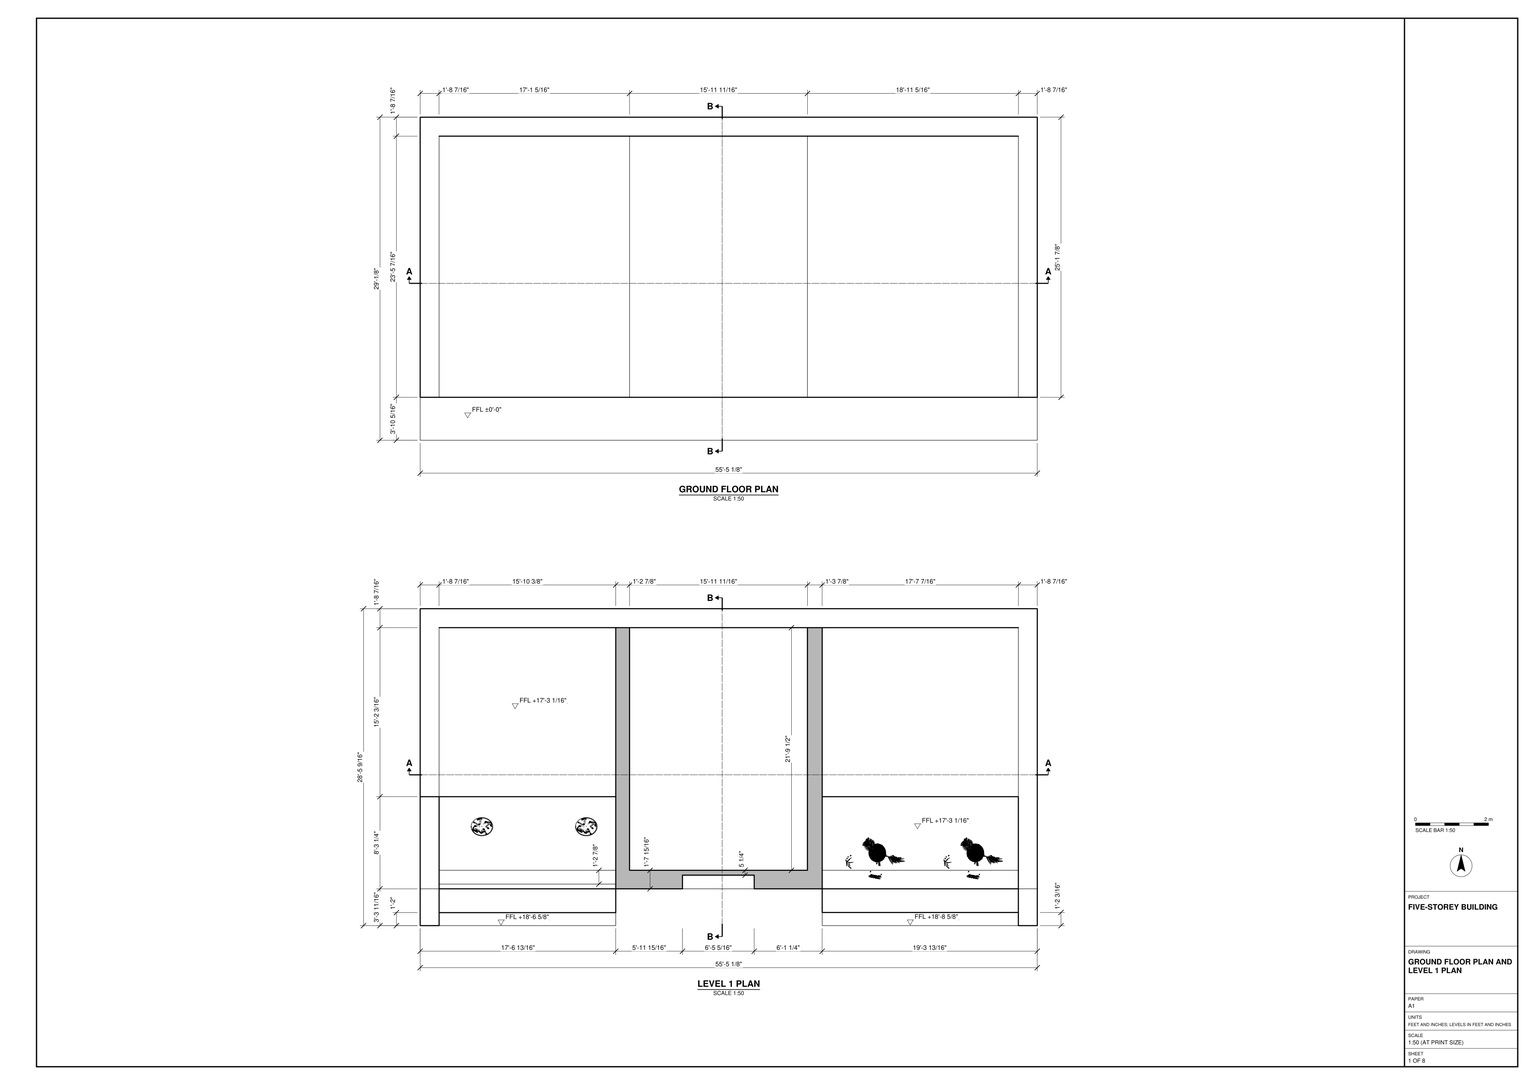
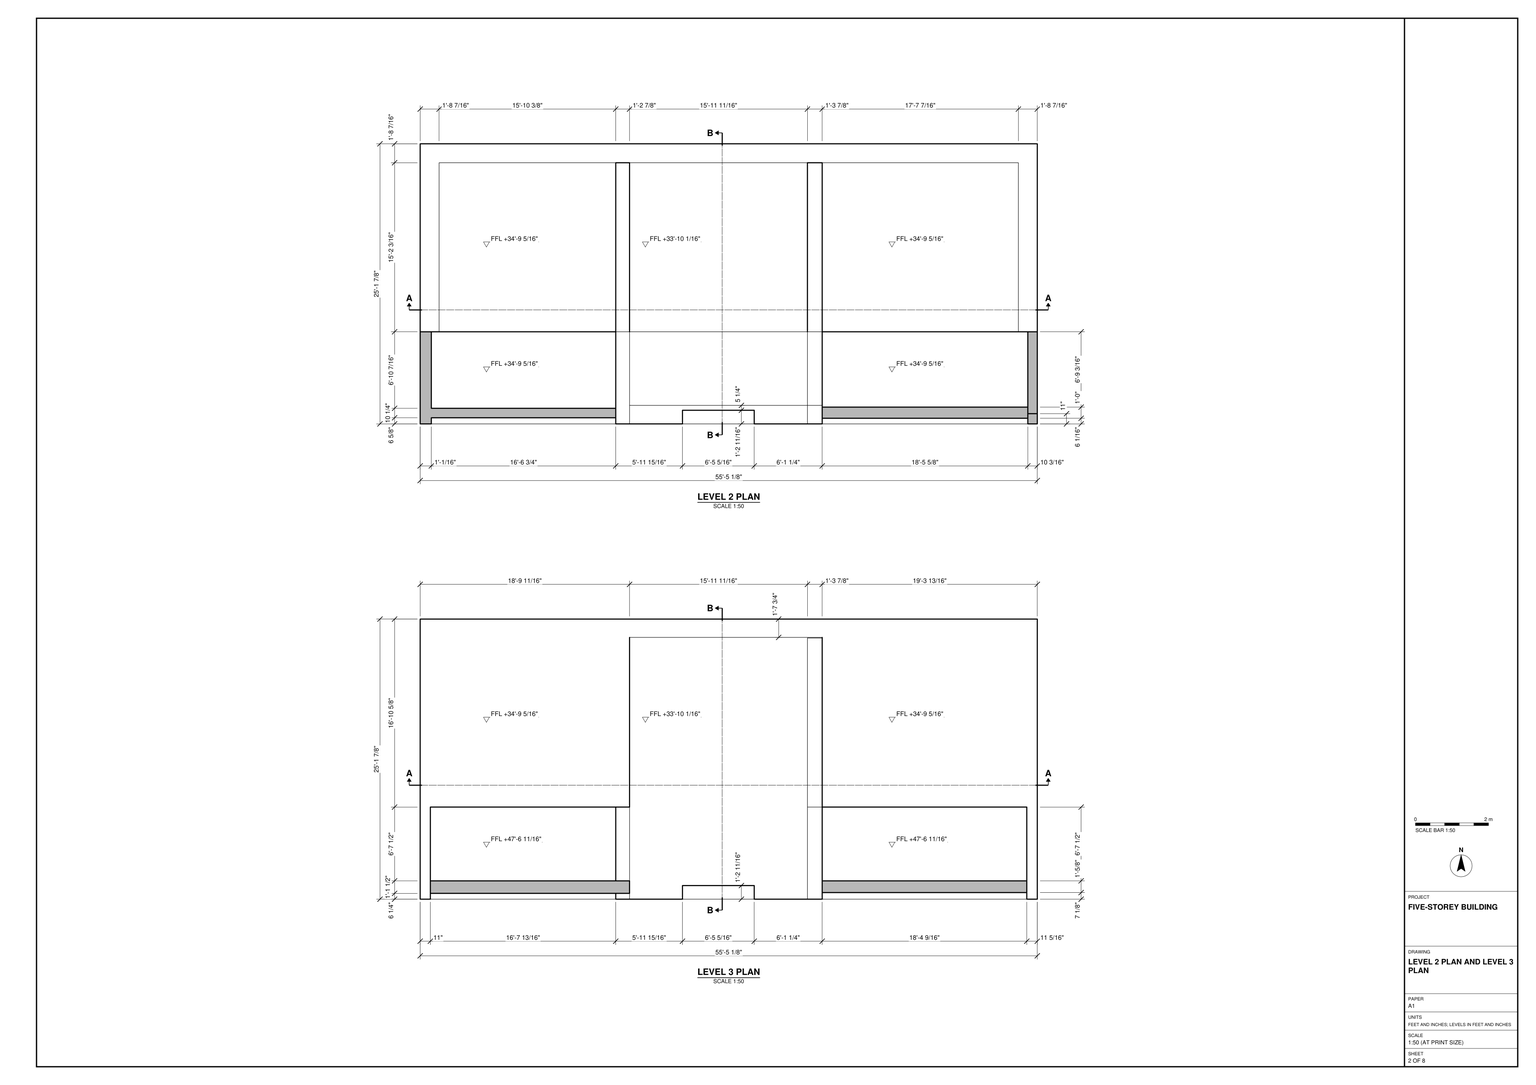
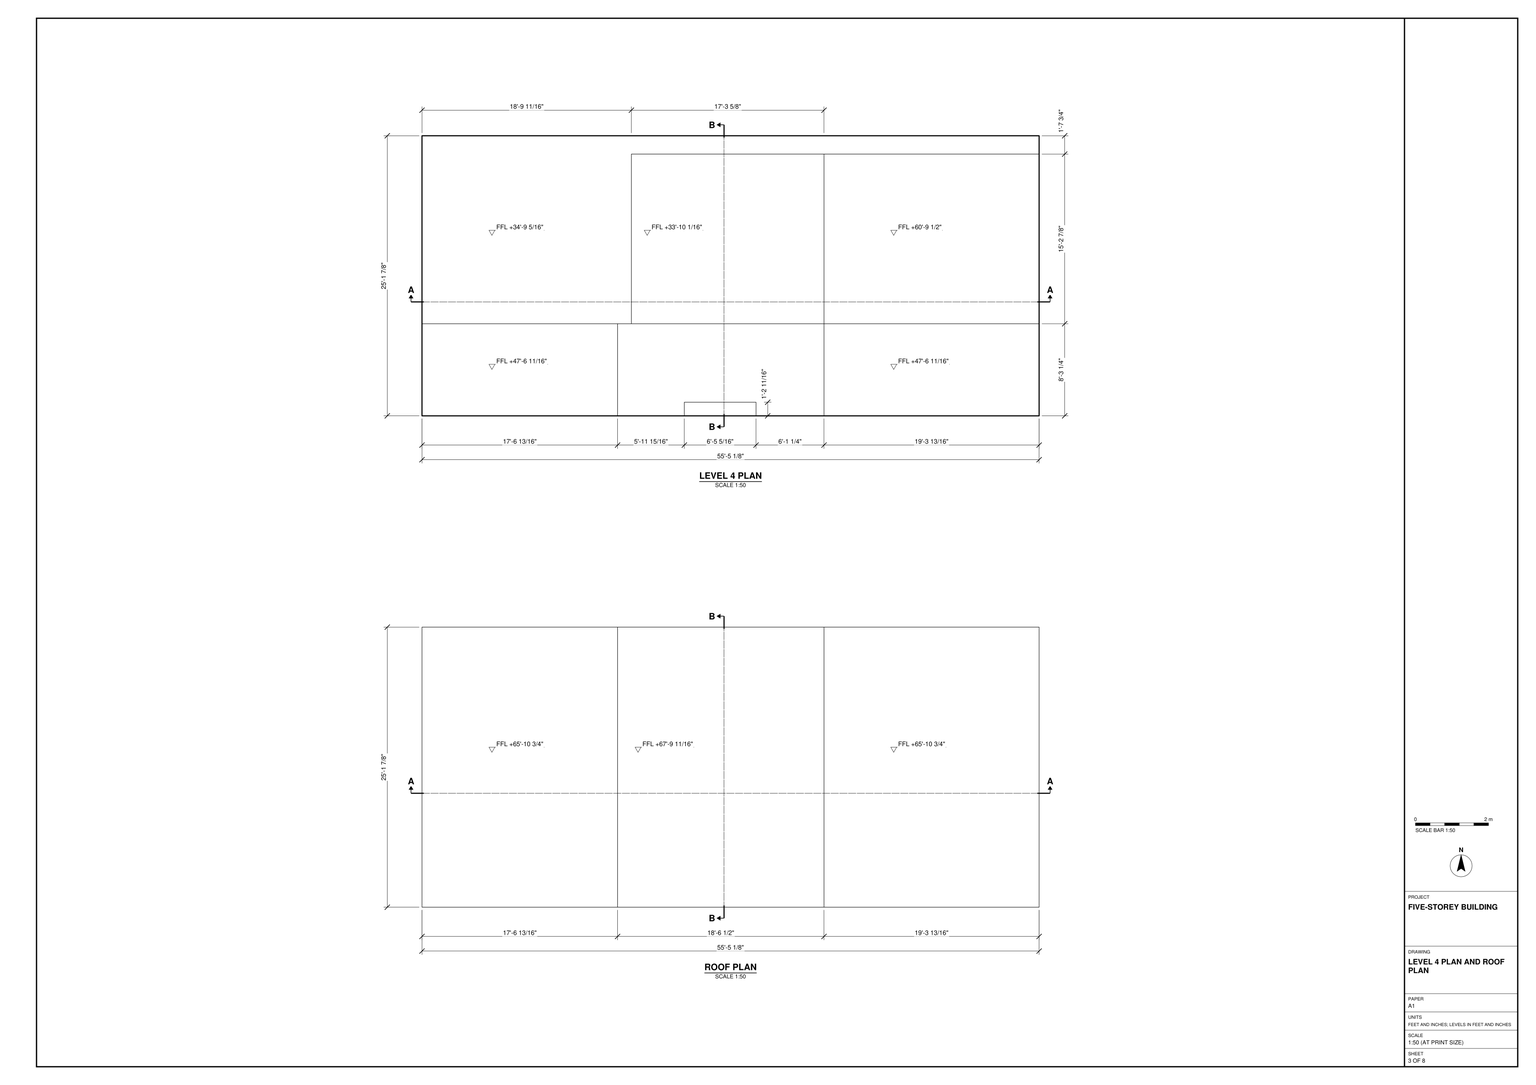
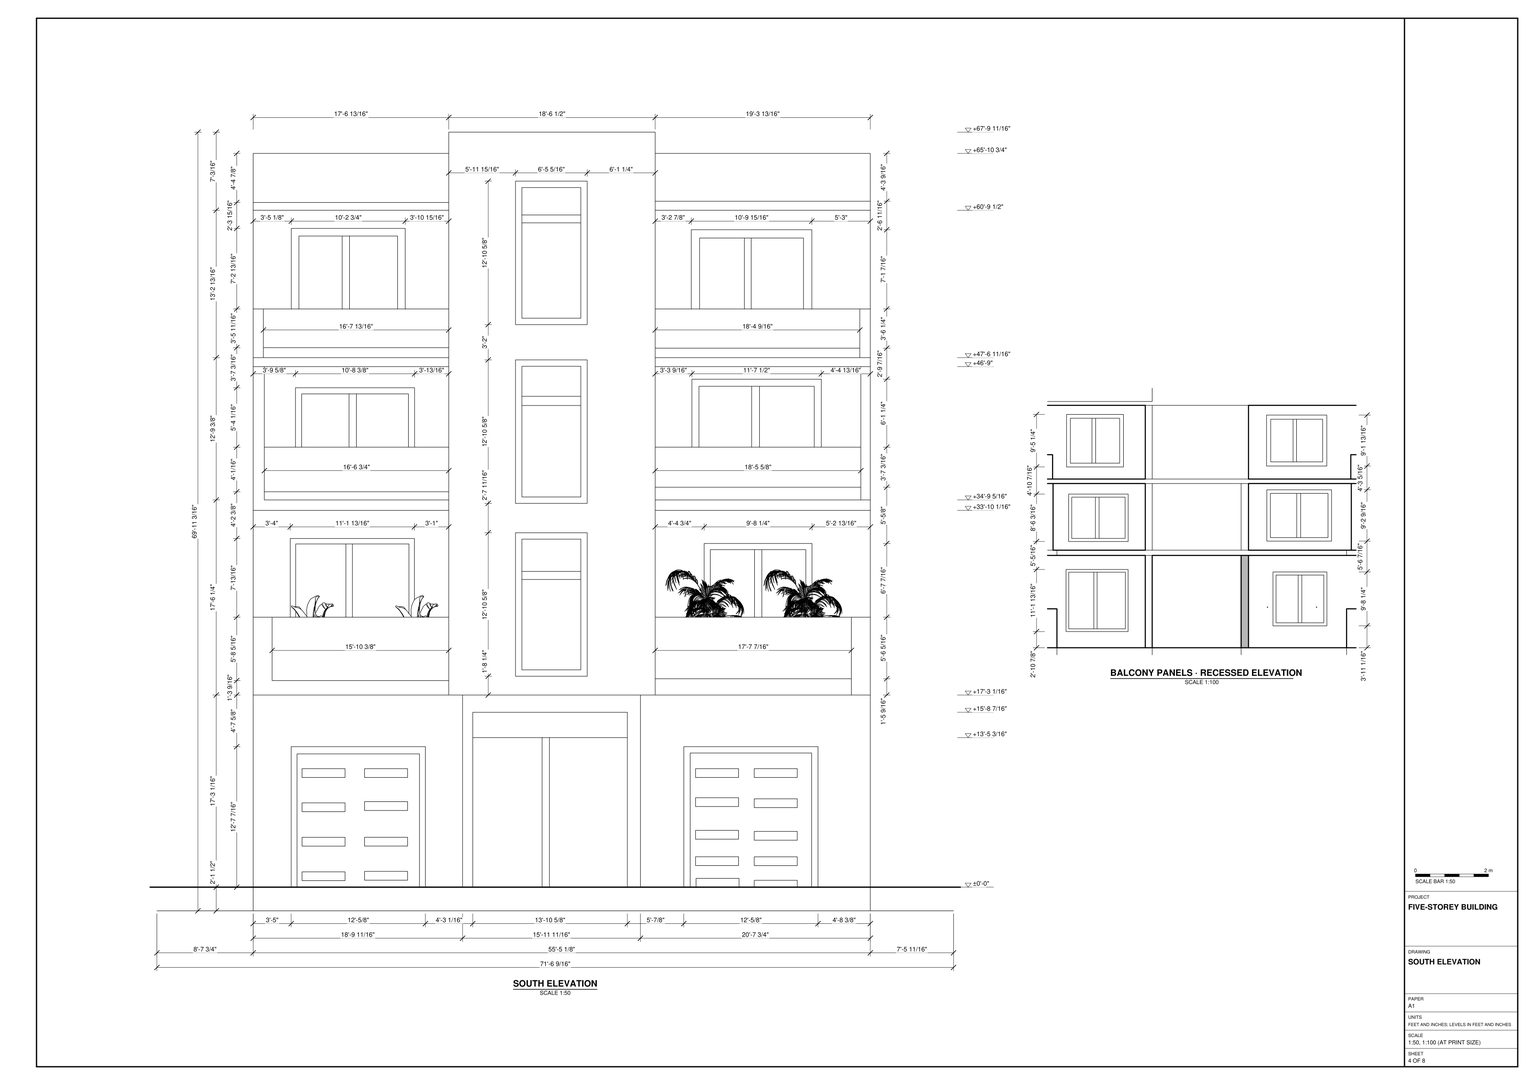
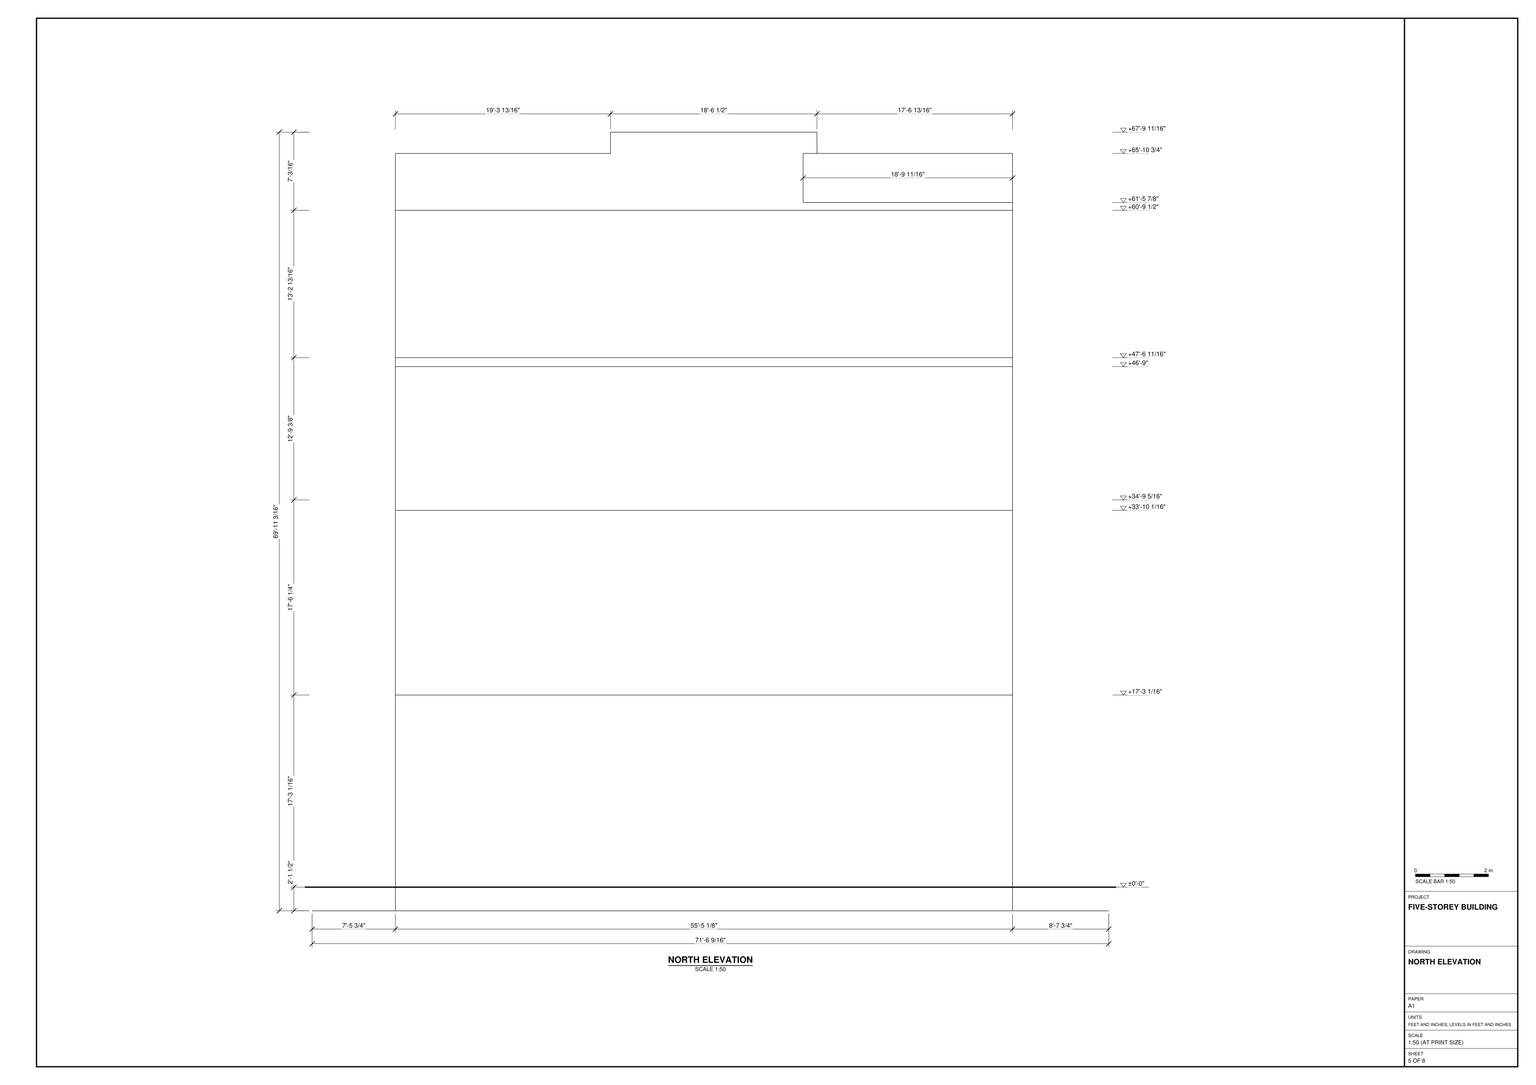
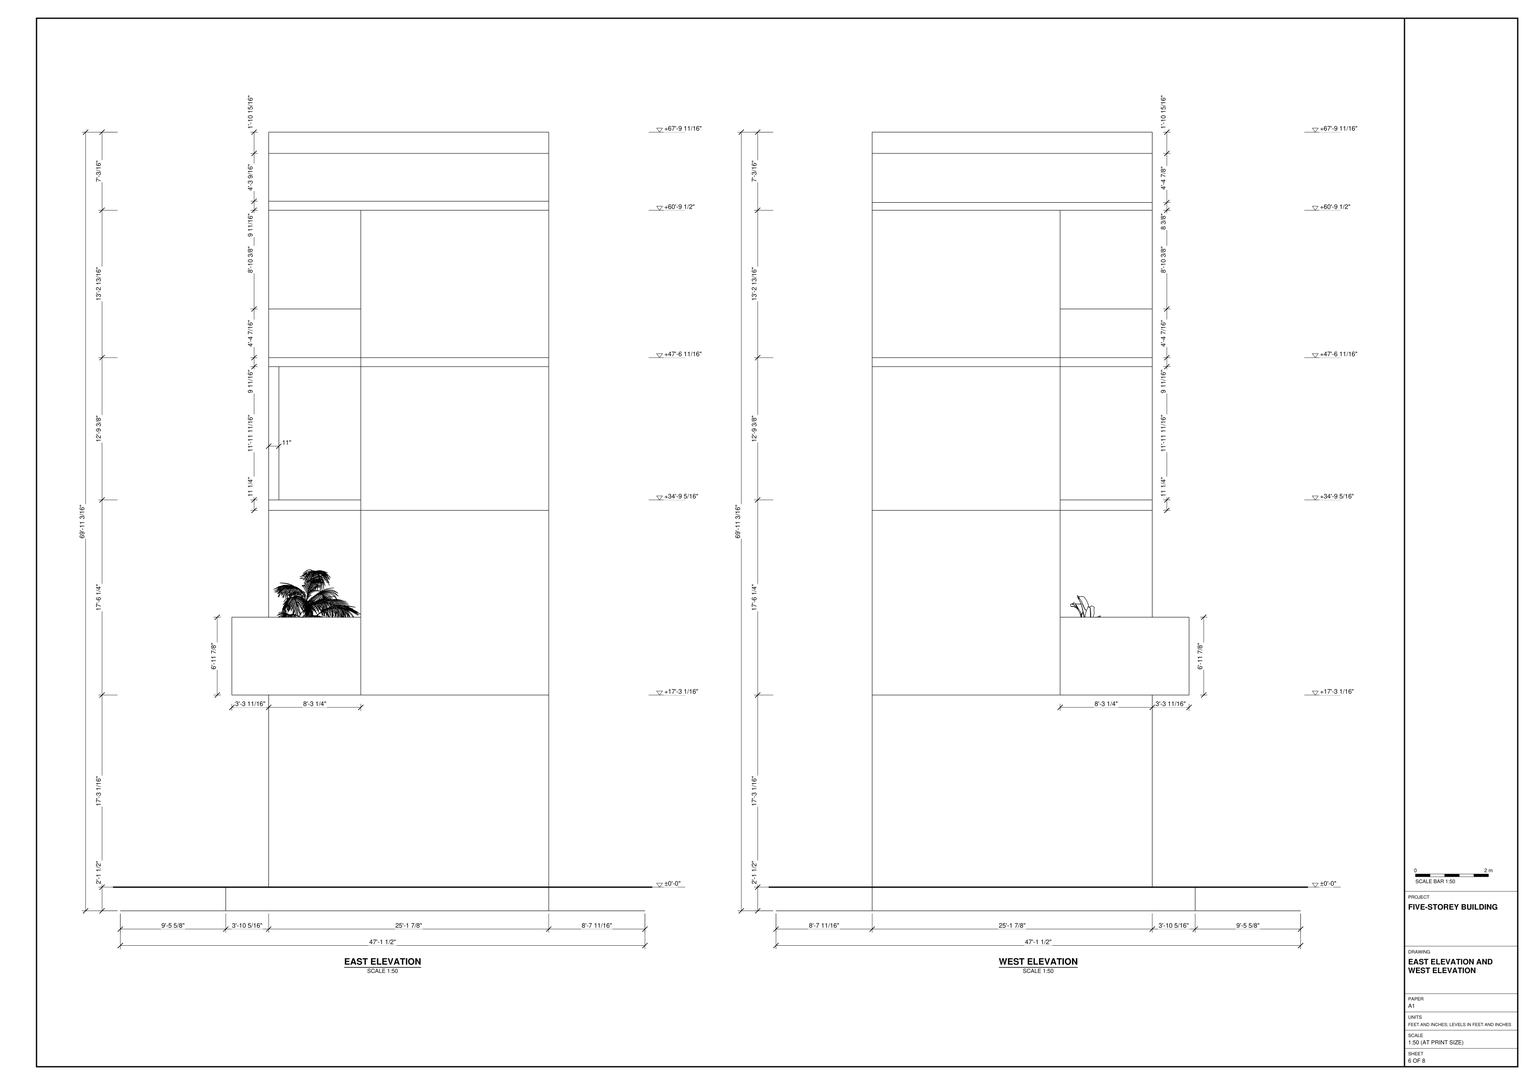
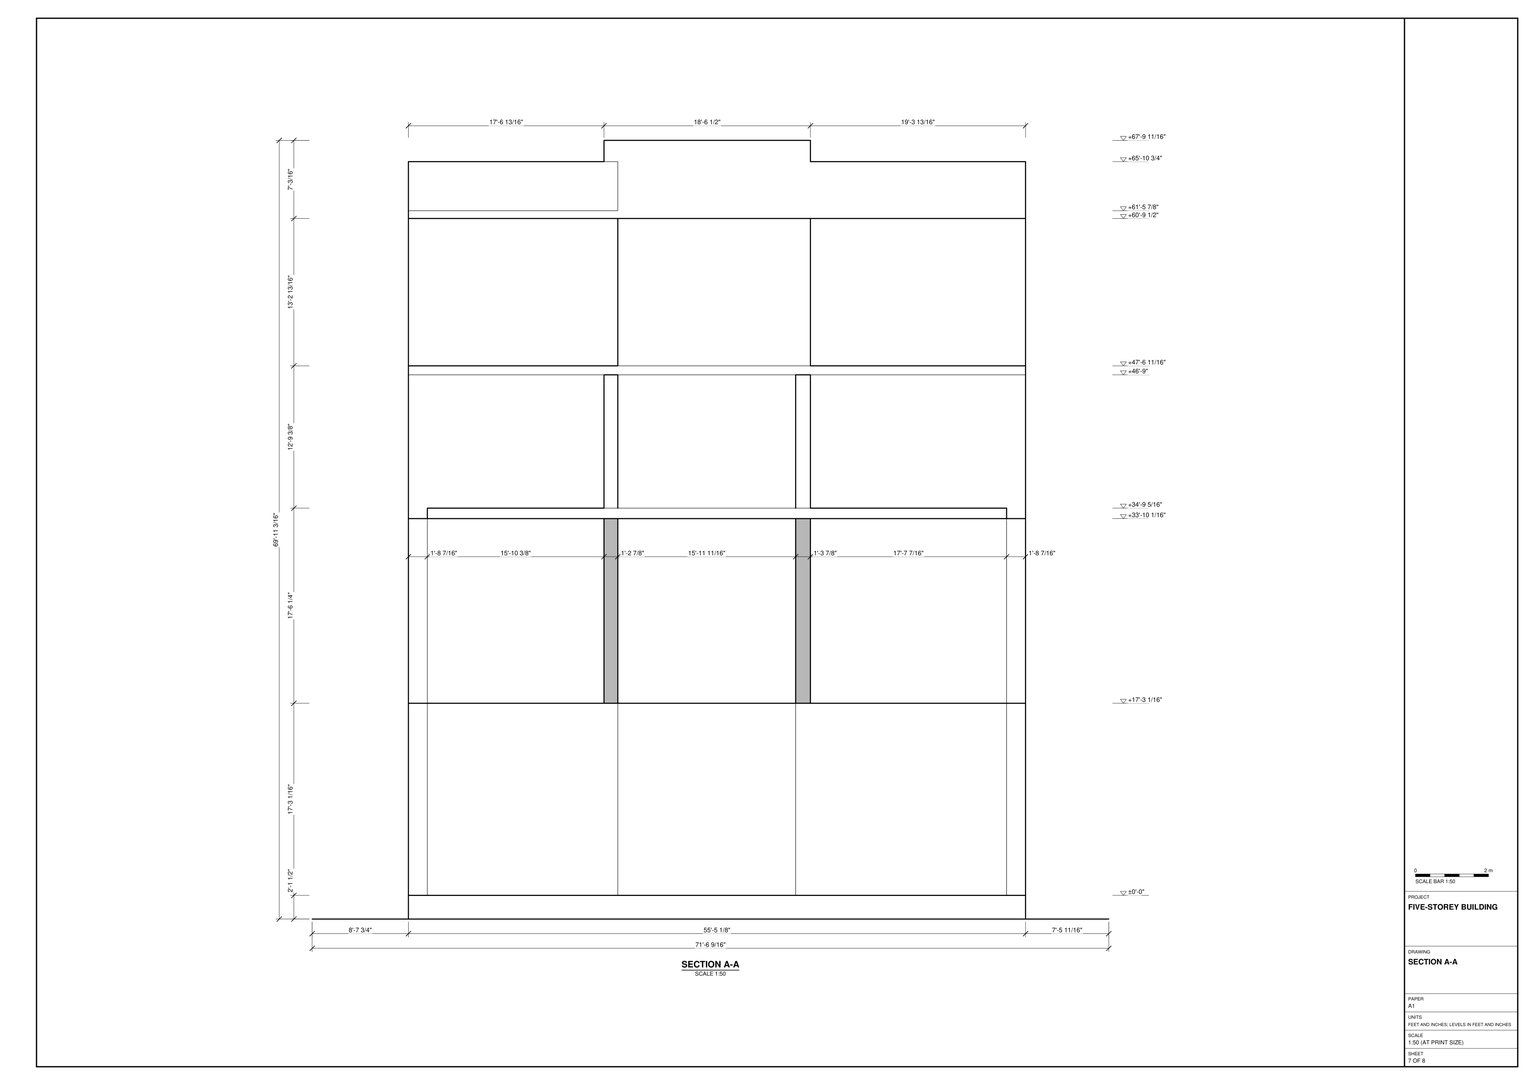
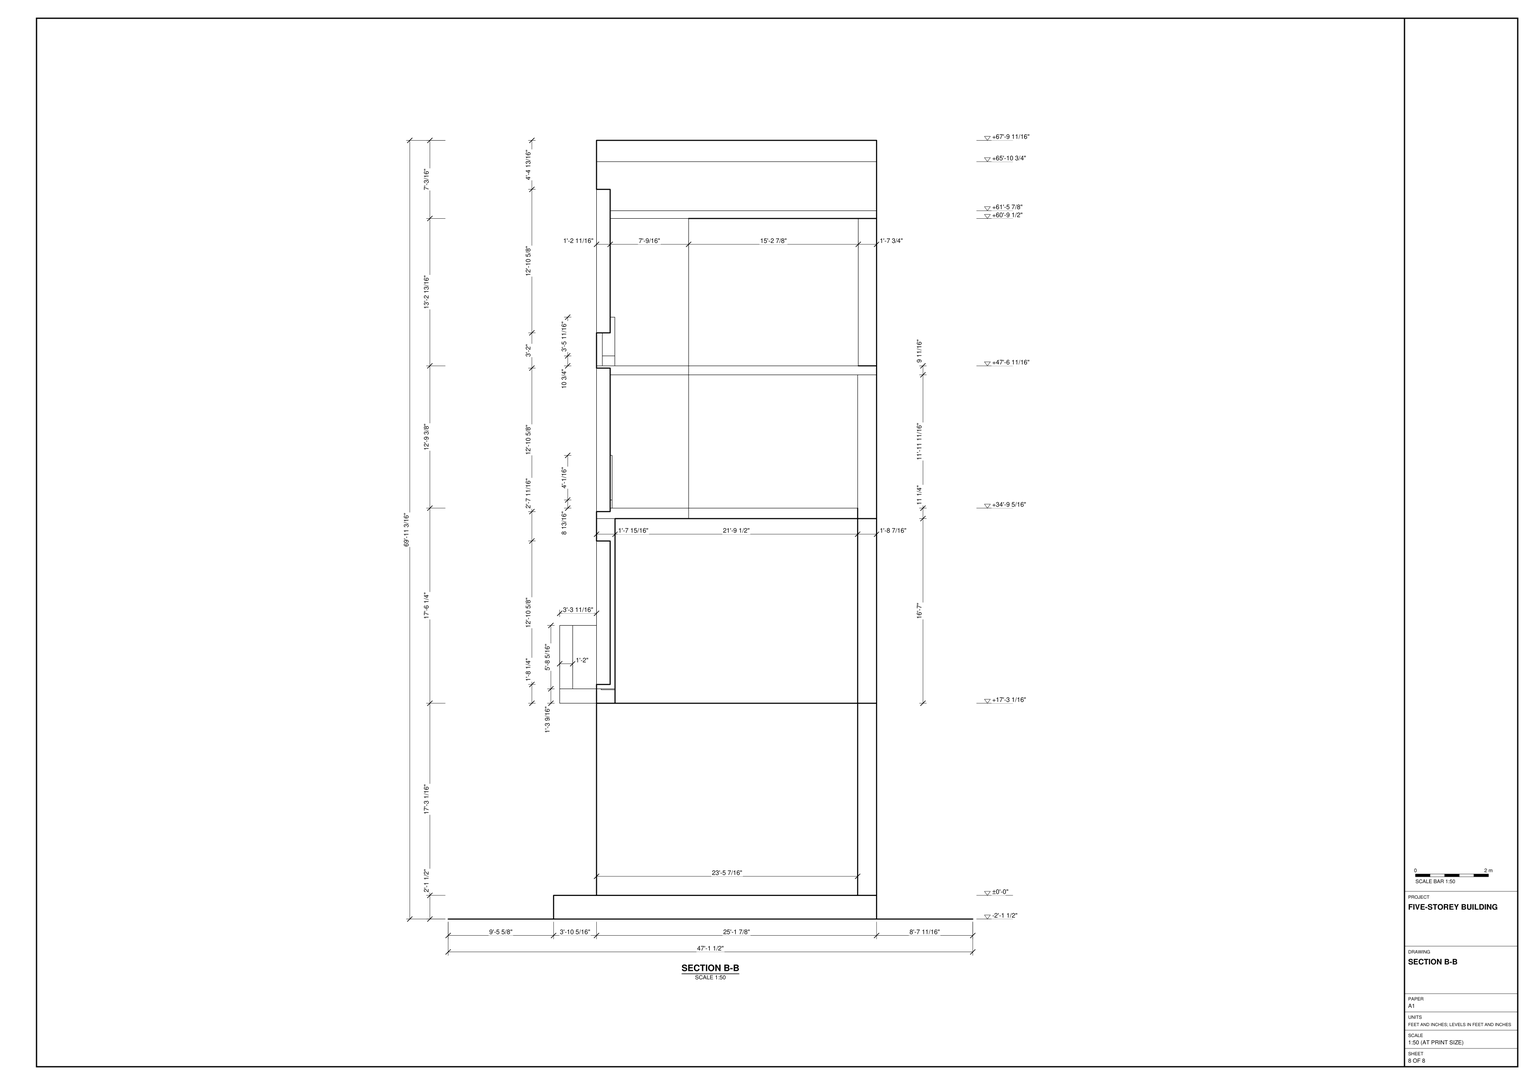
Build the five-storey building in SketchUp from task_files/diagram_01.pdf. Work in feet and inches. The overall model extents are 71'-6 9/16" along X, 47'-1 7/16" along Y and 69'-11 3/16" along Z. Use the dimensioned plans for the building footprint rather than treating the overall model extents as wall dimensions. Set the principal storey levels to ±0'-0", +17'-3 1/16", +34'-9 5/16", +47'-6 11/16" and +60'-9 1/2".

Lay out the three bays and the ground-floor strip that extends across their front. Model the perimeter and dividing walls at their drawn thicknesses. Follow the floor outlines and local changes in height in each bay rather than extending a full slab across every level. Include the recessed front edge of the central bay, the paired front platforms on Level 3 and the higher floor at the rear of the right bay on Level 4. Form the roof in three flat sections with the middle section raised. Follow the sheets for openings, stairs, built-in joinery and main furniture wherever shown. Decor and loose items, including the plants, may be any suitable library components.

Keep shell elements such as walls, slabs and roof sections, and each furniture or joinery piece, in separate groups or components. Use components for repeated parts. Save one SketchUp model as output_files/five_storey_stepped_building_with_raised_central_roof.skp.

# SketchUp Ruby script. Lengths in inches.
U = 1.inch
M = Sketchup.active_model
def pt(a) = Geom::Point3d.new(a.map { |v| v * U })
def face(e, loops, mat)
  f = e.add_face(loops[0].map { |a| pt(a) })
  loops[1..].each { |l| e.add_face(l.map { |a| pt(a) }).erase! }
  f.material = f.back_material = mat if mat
  f
end
# faces: each face lists its corners as indices into pts; further lists are holes
def faces(e, pts, list, mat = nil) = list.each { |f| face(e, (f[0].is_a?(Array) ? f : [f]).map { |l| l.map { |i| pts[i] } }, mat) }
# xy, xz, yz: faces in a plane at the given z, y or x. An outline is a flat list of corners, or four numbers for a rectangle; further outlines are holes
def ring(l) = l.size == 4 ? [[l[0], l[1]], [l[2], l[1]], [l[2], l[3]], [l[0], l[3]]] : l.each_slice(2).to_a
def flat(e, list, mat, &to3) = list.each { |f| face(e, (f[0].is_a?(Array) ? f : [f]).map { |l| ring(l).map { |u, v| to3.(u, v) } }, mat) }
def xy(e, z, list, mat = nil) = flat(e, list, mat) { |x, y| [x, y, z] }
def xz(e, y, list, mat = nil) = flat(e, list, mat) { |x, z| [x, y, z] }
def yz(e, x, list, mat = nil) = flat(e, list, mat) { |y, z| [x, y, z] }
def lines(e, pts, list) = list.each { |a, b| e.add_line(pt(pts[a]), pt(pts[b])) }
# prism: a flat outline (further loops are holes) pulled along v
def prism(e, loops, v, mat = nil)
  f = face(e, loops, mat); d = Geom::Vector3d.new(v.map { |x| x * U })
  f.pushpull(f.normal.samedirection?(d) ? d.length : -d.length)
end
def box(e, o, s, mat = nil) = prism(e, [[o, [o[0] + s[0], o[1], o[2]], [o[0] + s[0], o[1] + s[1], o[2]], [o[0], o[1] + s[1], o[2]]]], [0, 0, s[2]], mat)
def at(x, y, z, deg = 0) = Geom::Transformation.translation(pt([x, y, z])) * Geom::Transformation.rotation(ORIGIN, Z_AXIS, deg.degrees)
def axes(o, x, y, z) = Geom::Transformation.new([*x, 0, *y, 0, *z, 0, *pt(o).to_a, 1])
def part(name) = M.definitions.add(name)
# library, detail: a bought-in or finely detailed component or shape, given as its bounding box
def library(name, o, s) = part(name).tap { |d| box(d.entities, o, s) }
def detail(e, o, s) = box(e.add_group.entities, o, s)
def put(e, d, t, mat = nil) = e.add_instance(d, t).tap { |i| i.material = mat if mat }
def group(e, t, mat = nil) = e.add_group.tap { |g| g.transformation = t; g.material = mat if mat }.entities
root = M.entities
M.materials.add("[0012_Bisque]").color = [255, 228, 196]
M.materials.add("[0034_Wheat]").color = [245, 222, 179]
M.materials.add("[0035_Tan]").color = [191, 163, 127]
M.materials.add("[0035_Tan]1").color = [181, 155, 120]
M.materials.add("[0036_BurlyWood]").color = [222, 184, 135]
M.materials.add("[Carpet Diamond Olive]").color = [87, 77, 61]
M.materials.add("[Carpet Diamond Yellow]").color = [226, 217, 124]
M.materials.add("[Carpet Pattern Leaf Squares Tan]").color = [181, 154, 125]
M.materials.add("[Color M07]").color = [58, 58, 58]
M.materials.add("[Concrete Aggregate Smoke]").color = [154, 150, 148]
M.materials.add("[Field Square Tile]").color = [217, 201, 169]
M.materials.add("[Formica Graystone]").color = [149, 146, 135]
M.materials.add("[Formica Laminate Light]").color = [242, 214, 186]
M.materials.add("[Leather Red Brown]").color = [76, 40, 8]
M.materials.add("[Mirror 01]").color = [185, 185, 185]
M.materials.add("[Pavers Modular Brick]").color = [175, 143, 129]
M.materials.add("[Suede Blue]").color = [50, 57, 70]
M.materials.add("[Suede Dark Gray]").color = [85, 85, 85]
M.materials.add("[Terrazzo Tile Light]").color = [219, 217, 210]
M.materials.add("[Translucent Glass Gray]").color = [128, 128, 128]
M.materials["[Translucent Glass Gray]"].alpha = 0.5
M.materials.add("[Translucent Glass Safety]").color = [204, 235, 244]
M.materials["[Translucent Glass Safety]"].alpha = 0.5
M.materials.add("[Wallpaper Thin Brown Stripes]").color = [182, 160, 118]
M.materials.add("[Wood Floor Parquet]").color = [89, 54, 24]
M.materials.add("[Wood Floor Parquet]1").color = [104, 64, 28]
M.materials.add("[Wood Veneer 01]").color = [71, 41, 22]
c1 = library("Flora+17",[-57.52,158.6,-38.64],[66.99,62.88,77.28])
c2 = library("chau cay",[-24.34,-109.24,0],[56.46,62.58,79.69])
xy(root,-16.5,[[103.74,113.63,768.89,461.78]])
xy(root,-16.5,[[[0,0,858.59,565.46],[103.74,113.63,768.89,461.78]]],"[Pavers Modular Brick]")
xy(root,9,[[103.74,159.92,103.74,461.78,768.89,461.78,768.89,159.92,748.47,159.92,748.47,441.37,124.15,441.37,124.15,159.92],[124.15,159.92,329.44,441.37],[329.44,159.92,521.14,441.37],[521.14,159.92,748.47,441.37]])
xy(root,9,[[103.74,113.63,768.89,159.92]],"[Field Square Tile]")
xy(root,216.0625,[[103.74,159.92,124.15,259.18],[748.47,159.92,748.47,441.37,124.15,441.37,124.15,259.18,103.74,259.18,103.74,461.78,768.89,461.78,768.89,159.92],[124.15,159.92,314.56,179.87],[314.56,159.92,329.44,441.37],[329.44,159.92,521.14,179.87],
  [521.14,159.92,537.04,441.37],[537.04,159.92,748.47,179.87],[329.44,179.87,521.14,441.37],[124.15,259.18,314.56,441.37],[537.04,259.18,748.47,441.37]])
xy(root,216.0625,[[537.04,179.87,748.47,259.18]],"[Carpet Diamond Yellow]")
xy(root,216.0625,[[103.74,120.24,124.15,159.92],[124.15,120.24,314.56,159.92],[537.04,120.24,748.47,159.92],[748.47,120.24,768.89,159.92]],"[Formica Graystone]")
xy(root,216.0625,[[124.15,179.87,314.56,259.18]],"[Suede Blue]")
xy(root,230.625,[[124.15,164.98,314.56,179.87]])
xy(root,231.625,[[124.15,134.24,314.56,159.92],[124.15,159.92,314.56,164.98],[124.15,164.98,314.56,179.87]])
xy(root,231.625,[[124.15,120.24,314.56,134.24]],"[Formica Graystone]")
xy(root,233.625,[[537.04,134.42,748.47,159.92],[537.04,159.92,748.47,179.87]])
xy(root,233.625,[[537.04,120.24,748.47,134.42]],"[Formica Graystone]")
xy(root,236.31,[[386.47,159.92,463.79,174.61]],"[Formica Graystone]")
xy(root,299.9375,[[124.15,134.24,314.56,159.92],[537.04,134.42,748.47,159.92]])
xy(root,299.9375,[[103.74,120.24,124.15,259.18],[748.47,120.24,768.89,259.18]],"[Formica Graystone]")
xy(root,390.93,[[386.47,159.92,463.79,174.61]],"[Formica Graystone]")
xy(root,415.0625,[[103.74,159.92,314.56,259.18],[537.04,159.92,768.89,179.87],[329.44,179.87,521.14,259.18],[521.14,179.87,537.04,259.18],[537.04,179.87,768.89,259.18],
  [103.74,259.18,103.74,461.78,768.89,461.78,768.89,259.18,748.47,259.18,748.47,441.37,124.15,441.37,124.15,259.18],[124.15,259.18,314.56,441.37],[314.56,259.18,329.44,441.37],[329.44,259.18,521.14,441.37],[521.14,259.18,537.04,441.37],
  [537.04,259.18,748.47,441.37]])
xy(root,422.62,[[386.47,159.92,463.79,174.61]],"[Formica Graystone]")
xy(root,426.3125,[[758.68,159.92,768.89,170.93],[537.04,166,758.68,178.01],[124.15,166.53,314.56,176.75],[758.68,170.93,768.89,259.18],[124.15,259.18,314.56,441.37],
  [537.04,259.18,748.47,441.37]])
xy(root,426.3125,[[115.78,159.92,314.56,166.53],[537.04,159.92,758.68,166]],"[0012_Bisque]")
xy(root,426.3125,[[115.78,176.75,314.56,259.18]],"[Carpet Pattern Leaf Squares Tan]")
xy(root,426.3125,[[537.04,178.01,758.68,259.18]],"[Suede Dark Gray]")
xy(root,435.125,[[124.15,166.53,314.56,176.75]])
xy(root,440,[[537.04,166,758.68,178.01]])
xy(root,483.1875,[[537.04,166,758.68,178.01],[115.78,166.53,314.56,176.75]])
xy(root,570,[[103.74,159.92,115.78,259.18],[115.78,159.92,314.56,259.18],[537.04,159.92,758.68,259.18],[758.68,159.92,768.89,170.93],[758.68,170.93,768.89,259.18],
  [314.56,259.18,329.44,441.37],[521.14,259.18,537.04,441.37]])
xy(root,577.25,[[386.47,159.92,463.79,174.61]],"[Formica Graystone]")
xy(root,579.6875,[[103.74,159.92,103.74,461.78,768.89,461.78,768.89,159.92,757.58,159.92,757.58,259.18,537.04,259.18,537.04,442.04,329.44,442.04,329.44,259.18,114.73,259.18,114.73,159.92],[114.73,166.1875,329.44,179.67],[537.04,167.03,757.58,179.67]])
xy(root,579.6875,[[114.73,159.92,314.56,166.1875],[537.04,159.92,757.58,167.03]],"[0012_Bisque]")
xy(root,579.6875,[[114.73,179.67,314.56,259.18]],"[Carpet Diamond Olive]")
xy(root,579.6875,[[537.04,179.67,757.58,259.18]],"[Leather Red Brown]")
xy(root,589.875,[[537.04,167.03,757.58,179.67]])
xy(root,590.4375,[[114.73,166.1875,329.44,179.67]])
xy(root,615.25,[[386.47,159.92,463.79,174.61]],"[Formica Graystone]")
xy(root,632.125,[[114.73,166.1875,314.56,179.67],[314.56,166.1875,329.44,179.67],[537.04,167.03,757.58,179.67]])
xy(root,632.125,[[103.74,159.92,114.73,259.18],[757.58,159.92,768.89,259.18]],"[0012_Bisque]")
xy(root,738.5,[[103.74,159.92,314.56,259.18],[537.04,159.92,768.89,259.18],[103.74,259.18,103.74,461.78,768.89,461.78,768.89,442.04,329.44,442.04,329.44,259.18],[329.44,259.18,537.04,442.04],[537.04,259.18,768.89,442.04]])
xy(root,769.87,[[386.47,159.92,463.79,174.61]],"[Formica Graystone]")
xy(root,799.75,[[103.74,159.92,314.56,461.78],[537.04,159.92,768.89,461.78]],"[Concrete Aggregate Smoke]")
xy(root,822.6875,[[314.56,159.92,537.04,461.78]],"[Formica Laminate Light]")
xz(root,113.63,[[103.74,-16.5,768.89,9]],"[Field Square Tile]")
xz(root,120.24,[[103.74,216.0625,314.56,216.0625,314.56,231.625,124.15,231.625,124.15,299.9375,103.74,299.9375],[537.04,216.0625,748.47,233.625],[748.47,216.0625,768.89,299.9375]],"[Formica Graystone]")
xz(root,134.24,[[124.15,231.625,314.56,299.9375]],"[Translucent Glass Safety]")
xz(root,134.42,[[537.04,233.625,748.47,299.9375]],"[Translucent Glass Safety]")
xz(root,159.92,[[643.79,6.91,690.17,9]])
xz(root,159.92,[[103.74,415.0625,314.56,415.0625,314.56,426.3125,115.78,426.3125,115.78,570,103.74,570],[537.04,415.0625,768.89,426.3125],[758.68,426.3125,768.89,570],[103.74,570,314.56,579.6875],[537.04,570,768.89,579.6875],
  [103.74,579.6875,114.73,632.125],[757.58,579.6875,768.89,632.125]],"[0012_Bisque]")
xz(root,159.92,[[103.74,738.5,314.56,746.875],[537.04,738.5,768.89,748.22]],"[0034_Wheat]")
xz(root,159.92,[[103.74,9,144.73,9,144.73,160.4375,289.35,160.4375,289.35,9,329.44,9,329.44,216.0625,103.74,216.0625],[521.14,9,567.91,9,567.91,160.4375,712.54,160.4375,712.54,9,768.89,9,768.89,216.0625,521.14,216.0625]],"[0035_Tan]")
xz(root,159.92,[[581.08,9,627.45,18.5],[643.79,9,690.17,16.41],[156.42,16.03,202.79,25.53],[223.79,16.53,270.17,26.03],[643.79,32.22,690.17,41.72],
  [580.54,32.28,626.92,41.78],[156.42,53.22,202.79,62.72],[223.79,53.28,270.17,62.78],[643.79,59.6,690.17,69.1],[580.54,60.72,626.92,70.22],
  [156.42,90.35,202.79,99.85],[223.79,91.66,270.17,101.16],[643.79,94.72,690.17,104.22],[580.54,95.91,626.92,105.41],[156.42,127.22,202.79,136.72],
  [223.79,127.22,270.17,136.72],[580.54,127.22,626.92,136.72],[643.79,127.22,690.17,136.72]],"[0036_BurlyWood]")
xz(root,159.92,[[415.15,9,423.02,170.18],[340.42,170.18,507.04,197.4375]],"[Color M07]")
xz(root,159.92,[[103.74,746.875,314.56,799.75],[537.04,748.22,768.89,799.75]],"[Concrete Aggregate Smoke]")
xz(root,159.92,[[329.44,9,340.42,9,340.42,197.4375,507.04,197.4375,507.04,9,521.14,9,521.14,216.0625,329.44,216.0625],[[314.56,216.0625,537.04,822.6875],[386.47,615.25,463.79,769.87],[386.47,236.31,463.79,390.93],[386.47,422.62,463.79,577.25]]],"[Formica Laminate Light]")
xz(root,159.92,[[124.15,231.625,314.56,299.9375],[537.04,233.625,748.47,299.9375]],"[Translucent Glass Safety]")
xz(root,159.92,[[340.42,9,415.15,170.18],[423.02,9,507.04,170.18]],"[Wallpaper Thin Brown Stripes]")
xz(root,159.92,[[567.91,9,574.77,9,574.77,153.58,705.68,153.58,705.68,9,712.54,9,712.54,160.4375,567.91,160.4375],[[574.77,9,581.08,9,581.08,18.5,627.45,18.5,627.45,9,643.79,9,643.79,16.41,690.17,16.41,690.17,9,705.68,9,705.68,153.58,574.77,153.58],[580.54,95.91,626.92,105.41],[580.54,60.72,626.92,70.22],[580.54,32.28,626.92,41.78],[580.54,127.22,626.92,136.72],[643.79,127.22,690.17,136.72],[643.79,94.72,690.17,104.22],[643.79,59.6,690.17,69.1],[643.79,32.22,690.17,41.72]]],"[Wood Floor Parquet]")
xz(root,159.92,[[144.73,9,151.01,9,151.01,152.625,283.01,152.625,283.01,9,289.35,9,289.35,160.4375,144.73,160.4375],[[151.01,9,283.01,152.625],[156.42,127.22,202.79,136.72],[223.79,127.22,270.17,136.72],[156.42,90.35,202.79,99.85],[156.42,53.22,202.79,62.72],[156.42,16.03,202.79,25.53],[223.79,91.66,270.17,101.16],[223.79,53.28,270.17,62.78],[223.79,16.53,270.17,26.03]]],"[Wood Floor Parquet]1")
xz(root,164.98,[[124.15,230.625,314.56,231.625]])
xz(root,166,[[537.04,426.3125,758.68,440]],"[0012_Bisque]")
xz(root,166,[[537.04,440,758.68,483.1875]],"[Translucent Glass Safety]")
xz(root,166.1875,[[314.56,579.6875,329.44,590.4375],[314.56,590.4375,329.44,632.125]])
xz(root,166.1875,[[114.73,579.6875,314.56,590.4375]],"[0012_Bisque]")
xz(root,166.1875,[[114.73,590.4375,314.56,632.125]],"[Translucent Glass Safety]")
xz(root,166.53,[[115.78,426.3125,314.56,435.125]],"[0012_Bisque]")
xz(root,166.53,[[115.78,435.125,314.56,483.1875]],"[Translucent Glass Safety]")
xz(root,167.03,[[537.04,579.6875,757.58,589.875]],"[0012_Bisque]")
xz(root,167.03,[[537.04,589.875,757.58,632.125]],"[Translucent Glass Safety]")
xz(root,170.93,[[758.68,426.3125,768.89,570]])
xz(root,174.61,[[[386.47,236.31,463.79,390.93],[393.37,243.21,456.89,384.04]],[393.37,340.6,456.89,349.29],[[386.47,422.62,463.79,577.25],[393.37,429.52,456.89,570.35]],[393.37,528.08,456.89,537.95],[[386.47,615.25,463.79,769.87],[393.37,622.14,456.89,762.97]],
  [393.37,724.95,456.89,733.42]],"[Terrazzo Tile Light]")
xz(root,174.61,[[393.37,243.21,456.89,340.6],[393.37,349.29,456.89,384.04],[393.37,429.52,456.89,528.08],[393.37,537.95,456.89,570.35],[393.37,622.14,456.89,724.95],
  [393.37,733.42,456.89,762.97]],"[Translucent Glass Gray]")
xz(root,176.75,[[115.78,426.3125,124.15,435.125],[124.15,426.3125,314.56,435.125]])
xz(root,176.75,[[115.78,435.125,314.56,483.1875]],"[Translucent Glass Safety]")
xz(root,178.01,[[537.04,426.3125,758.68,440]])
xz(root,178.01,[[537.04,440,758.68,483.1875]],"[Translucent Glass Safety]")
xz(root,179.67,[[114.73,579.6875,314.56,590.4375],[314.56,579.6875,329.44,590.4375],[537.04,579.6875,757.58,589.875],[314.56,590.4375,329.44,632.125]])
xz(root,179.67,[[537.04,589.875,757.58,632.125],[114.73,590.4375,314.56,632.125]],"[Translucent Glass Safety]")
xz(root,179.87,[[124.15,216.0625,314.56,230.625],[329.44,216.0625,521.14,415.0625],[537.04,216.0625,748.47,233.625],[124.15,230.625,314.56,231.625]])
xz(root,259.18,[[103.74,216.0625,124.15,299.9375],[103.74,415.0625,124.15,426.3125],[748.47,415.0625,768.89,426.3125],[103.74,426.3125,115.78,570],[758.68,426.3125,768.89,570],
  [314.56,579.6875,329.44,738.5]])
xz(root,259.18,[[[124.15,216.0625,314.56,216.0625,314.56,415.0625,103.74,415.0625,103.74,299.9375,124.15,299.9375],[143.72,250.95,277.53,384.76]],[[537.04,216.0625,748.47,216.0625,748.47,299.9375,768.89,299.9375,768.89,415.0625,537.04,415.0625],[589.81,263.15,706.06,379.4]],[[115.78,426.3125,314.56,570],[149.35,445.04,277.72,547.23]],[[537.04,426.3125,758.68,570],[576.59,445.86,716.09,556.43]],[[114.73,579.6875,314.56,579.6875,314.56,738.5,103.74,738.5,103.74,632.125,114.73,632.125],[144.84,605.68,267.59,718.93]],
  [[537.04,579.6875,757.58,579.6875,757.58,632.125,768.89,632.125,768.89,738.5,537.04,738.5],[575.94,607.73,705.88,717.54]]],"[0035_Tan]1")
xz(root,259.18,[[149.59,256.82,203.69,378.89],[210.73,256.82,271.66,378.89],[596.47,269.81,644.14,372.74],[652.01,269.81,699.4,372.74]],"[Mirror 01]")
xz(root,259.18,[[155.99,451.69,207.06,540.58],[215,451.69,271.07,540.58],[584.22,453.49,641.02,548.8],[649.47,453.49,708.46,548.8],[153.07,613.91,199.67,710.71],
  [207.57,613.91,259.37,710.71],[584.91,616.7,633.1875,708.57],[640.53,616.7,696.91,708.57]],"[Translucent Glass Gray]")
xz(root,259.18,[[[143.72,250.95,277.53,384.76],[149.59,256.82,271.66,378.89]],[203.69,256.82,210.73,378.89],[[589.81,263.15,706.06,379.4],[596.47,269.81,699.4,372.74]],[644.14,269.81,652.01,372.74],[[149.35,445.04,277.72,547.23],[155.99,451.69,271.07,540.58]],
  [[576.59,445.86,716.09,556.43],[584.22,453.49,708.46,548.8]],[207.06,451.69,215,540.58],[641.02,453.49,649.47,548.8],[[144.84,605.68,267.59,718.93],[153.07,613.91,259.37,710.71]],[[575.94,607.73,705.88,717.54],[584.91,616.7,696.91,708.57]],
  [199.67,613.91,207.57,710.71],[633.1875,616.7,640.53,708.57]],"[Wood Veneer 01]")
xz(root,441.37,[[124.15,9,329.44,216.0625],[329.44,9,521.14,216.0625],[521.14,9,748.47,216.0625],[124.15,216.0625,314.56,415.0625],[314.56,216.0625,329.44,415.0625],
  [329.44,216.0625,521.14,415.0625],[521.14,216.0625,537.04,415.0625],[537.04,216.0625,748.47,415.0625],[124.15,415.0625,748.47,426.3125],[314.56,426.3125,329.44,570],
  [521.14,426.3125,537.04,570]])
xz(root,461.78,[[103.74,9,768.89,216.0625]],"[0035_Tan]")
xz(root,461.78,[[103.74,216.0625,768.89,415.0625],[103.74,415.0625,768.89,570],[103.74,570,768.89,579.6875],[103.74,579.6875,768.89,738.5]],"[0035_Tan]1")
xz(root,461.78,[[103.74,738.5,103.74,746.875,329.44,746.875,329.44,799.75,314.56,799.75,314.56,822.6875,537.04,822.6875,537.04,799.75,768.89,799.75,768.89,738.5],[103.74,746.875,329.44,799.75]],"[Concrete Aggregate Smoke]")
xz(root,461.78,[[103.74,-16.5,768.89,9]],"[Field Square Tile]")
yz(root,103.74,[[159.92,579.6875,259.18,632.125]],"[0012_Bisque]")
yz(root,103.74,[[159.92,738.5,461.78,746.875]],"[0034_Wheat]")
yz(root,103.74,[[159.92,9,461.78,216.0625]],"[0035_Tan]")
yz(root,103.74,[[259.18,216.0625,461.78,415.0625],[159.92,415.0625,259.18,426.3125],[259.18,415.0625,461.78,570],[159.92,426.3125,259.18,570],[159.92,570,259.18,579.6875],
  [259.18,570,461.78,579.6875],[259.18,579.6875,461.78,738.5]],"[0035_Tan]1")
yz(root,103.74,[[159.92,746.875,461.78,799.75]],"[Concrete Aggregate Smoke]")
yz(root,103.74,[[113.63,-16.5,461.78,9]],"[Field Square Tile]")
yz(root,103.74,[[120.24,216.0625,259.18,299.9375]],"[Formica Graystone]")
yz(root,114.73,[[166.1875,579.6875,179.67,590.4375],[166.1875,590.4375,179.67,632.125]])
yz(root,114.73,[[159.92,579.6875,166.1875,632.125],[179.67,579.6875,259.18,632.125]],"[0012_Bisque]")
yz(root,115.78,[[159.92,426.3125,166.53,426.3125,166.53,483.1875,176.75,483.1875,176.75,426.3125,259.18,426.3125,259.18,570,159.92,570]],"[0035_Tan]1")
yz(root,124.15,[[164.98,230.625,179.87,231.625],[134.24,231.625,159.92,299.9375],[259.18,415.0625,441.37,426.3125]])
yz(root,124.15,[[179.87,216.0625,259.18,216.0625,259.18,299.9375,159.92,299.9375,159.92,231.625,179.87,231.625],[120.24,231.625,134.24,299.9375]],"[Formica Graystone]")
yz(root,314.56,[[159.92,216.0625,159.92,231.625,164.98,231.625,164.98,230.625,179.87,230.625,179.87,216.0625],[259.18,216.0625,441.37,415.0625],[164.98,230.625,179.87,231.625],[166.53,426.3125,176.75,435.125],[259.18,426.3125,441.37,570],
  [166.53,435.125,176.75,483.1875]])
yz(root,314.56,[[179.87,216.0625,179.87,231.625,159.92,231.625,159.92,415.0625,259.18,415.0625,259.18,216.0625],[159.92,426.3125,159.92,570,259.18,570,259.18,426.3125,176.75,426.3125,176.75,483.1875,166.53,483.1875,166.53,426.3125],[159.92,579.6875,159.92,738.5,259.18,738.5,259.18,579.6875,179.67,579.6875,179.67,632.125,166.1875,632.125,166.1875,579.6875]],"[0035_Tan]1")
yz(root,314.56,[[120.24,216.0625,159.92,231.625]],"[Formica Graystone]")
yz(root,314.56,[[159.92,799.75,461.78,822.6875]],"[Formica Laminate Light]")
yz(root,314.56,[[134.24,231.625,159.92,299.9375]],"[Translucent Glass Safety]")
yz(root,329.44,[[179.87,216.0625,441.37,415.0625],[259.18,426.3125,441.37,570],[166.1875,579.6875,179.67,590.4375],[259.18,579.6875,442.04,738.5],[166.1875,590.4375,179.67,632.125]])
yz(root,386.47,[[159.92,236.31,174.61,390.93],[159.92,422.62,174.61,577.25],[159.92,615.25,174.61,769.87]],"[Formica Graystone]")
yz(root,463.79,[[159.92,236.31,174.61,390.93],[159.92,422.62,174.61,577.25],[159.92,615.25,174.61,769.87]],"[Formica Graystone]")
yz(root,521.14,[[179.87,216.0625,441.37,415.0625],[259.18,426.3125,441.37,570]])
yz(root,537.04,[[159.92,216.0625,179.87,233.625],[259.18,216.0625,441.37,415.0625],[166,426.3125,178.01,440],[259.18,426.3125,441.37,570],[166,440,178.01,483.1875],
  [167.03,579.6875,179.67,589.875],[259.18,579.6875,442.04,738.5],[167.03,589.875,179.67,632.125]])
yz(root,537.04,[[179.87,216.0625,259.18,216.0625,259.18,415.0625,159.92,415.0625,159.92,233.625,179.87,233.625],[159.92,426.3125,166,426.3125,166,483.1875,178.01,483.1875,178.01,426.3125,259.18,426.3125,259.18,570,159.92,570],[159.92,579.6875,167.03,579.6875,167.03,632.125,179.67,632.125,179.67,579.6875,259.18,579.6875,259.18,738.5,159.92,738.5]],"[0035_Tan]1")
yz(root,537.04,[[120.24,216.0625,159.92,233.625]],"[Formica Graystone]")
yz(root,537.04,[[159.92,799.75,461.78,822.6875]],"[Formica Laminate Light]")
yz(root,537.04,[[134.42,233.625,159.92,299.9375]],"[Translucent Glass Safety]")
yz(root,748.47,[[120.24,216.0625,179.87,233.625],[134.42,233.625,159.92,299.9375],[259.18,415.0625,441.37,426.3125]])
yz(root,748.47,[[179.87,216.0625,179.87,233.625,159.92,233.625,159.92,299.9375,259.18,299.9375,259.18,216.0625],[120.24,233.625,134.42,299.9375]],"[Formica Graystone]")
yz(root,757.58,[[167.03,579.6875,179.67,589.875],[167.03,589.875,179.67,632.125]])
yz(root,757.58,[[159.92,579.6875,167.03,632.125],[179.67,579.6875,259.18,632.125]],"[0012_Bisque]")
yz(root,758.68,[[166,426.3125,170.93,440],[170.93,426.3125,178.01,440],[166,440,170.93,483.1875],[170.93,440,178.01,483.1875]])
yz(root,758.68,[[159.92,426.3125,159.92,570,170.93,570,170.93,483.1875,166,483.1875,166,426.3125]],"[0012_Bisque]")
yz(root,758.68,[[178.01,426.3125,178.01,483.1875,170.93,483.1875,170.93,570,259.18,570,259.18,426.3125]],"[0035_Tan]1")
yz(root,768.89,[[159.92,579.6875,259.18,632.125]],"[0012_Bisque]")
yz(root,768.89,[[159.92,738.5,461.78,748.22]],"[0034_Wheat]")
yz(root,768.89,[[159.92,9,461.78,216.0625]],"[0035_Tan]")
yz(root,768.89,[[259.18,216.0625,461.78,415.0625],[159.92,415.0625,259.18,426.3125],[259.18,415.0625,461.78,570],[159.92,426.3125,170.93,570],[170.93,426.3125,259.18,570],
  [159.92,570,259.18,579.6875],[259.18,570,461.78,579.6875],[259.18,579.6875,461.78,738.5]],"[0035_Tan]1")
yz(root,768.89,[[159.92,748.22,461.78,799.75]],"[Concrete Aggregate Smoke]")
yz(root,768.89,[[113.63,-16.5,461.78,9]],"[Field Square Tile]")
yz(root,768.89,[[120.24,216.0625,259.18,299.9375]],"[Formica Graystone]")
p = [[329.44,179.87,415.0625],[329.44,159.92,415.0625],[521.14,179.87,415.0625],[521.14,159.92,415.0625],[329.44,259.18,426.3125],[329.44,159.92,426.3125],
  [521.14,259.18,570],[521.14,159.92,570],[329.44,259.18,570],[329.44,159.92,570]]
lines(root,p,[[0,1],[2,3],[4,5],[6,7],[8,9]])
put(root,c1,axes([629.4,-73.04,292.38],[1.41,0,0],[0,1.5,0],[0,0,1.52064]))
put(root,c1,axes([735.11,-73.04,292.38],[1.41,0,0],[0,1.5,0],[0,0,1.52064]))
put(root,c2,axes([168.26,305.84,216.0625],[1.19,0,0],[0,1,0],[0,0,1.4518]))
put(root,c2,axes([280.76,305.84,216.0625],[1.19,0,0],[0,1,0],[0,0,1.4518]))
